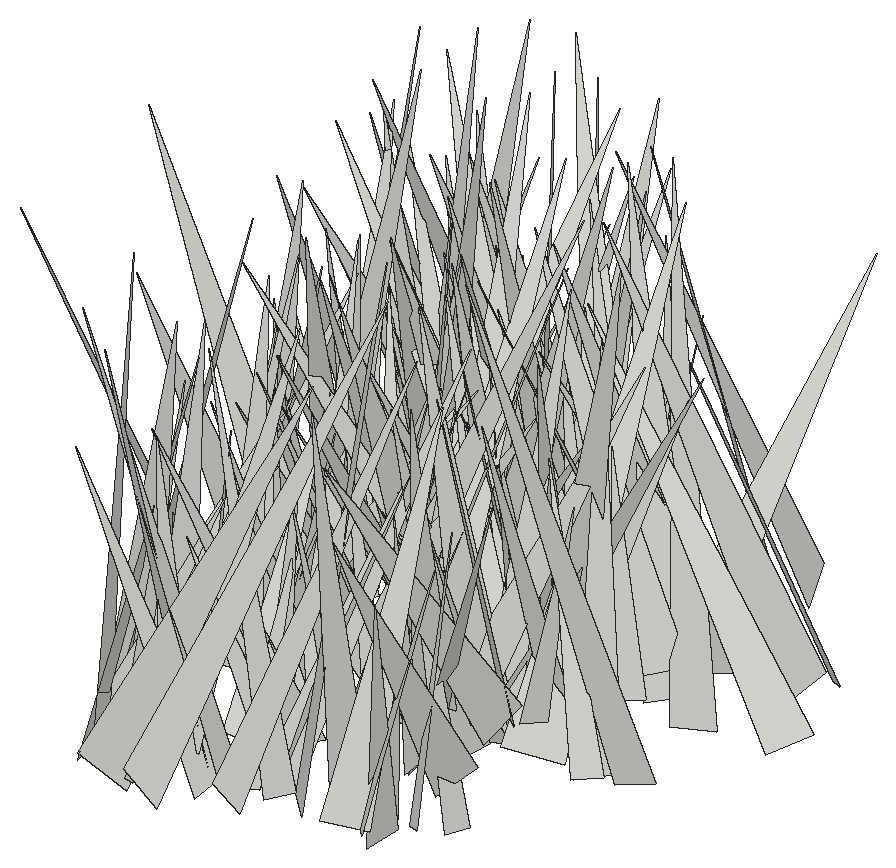
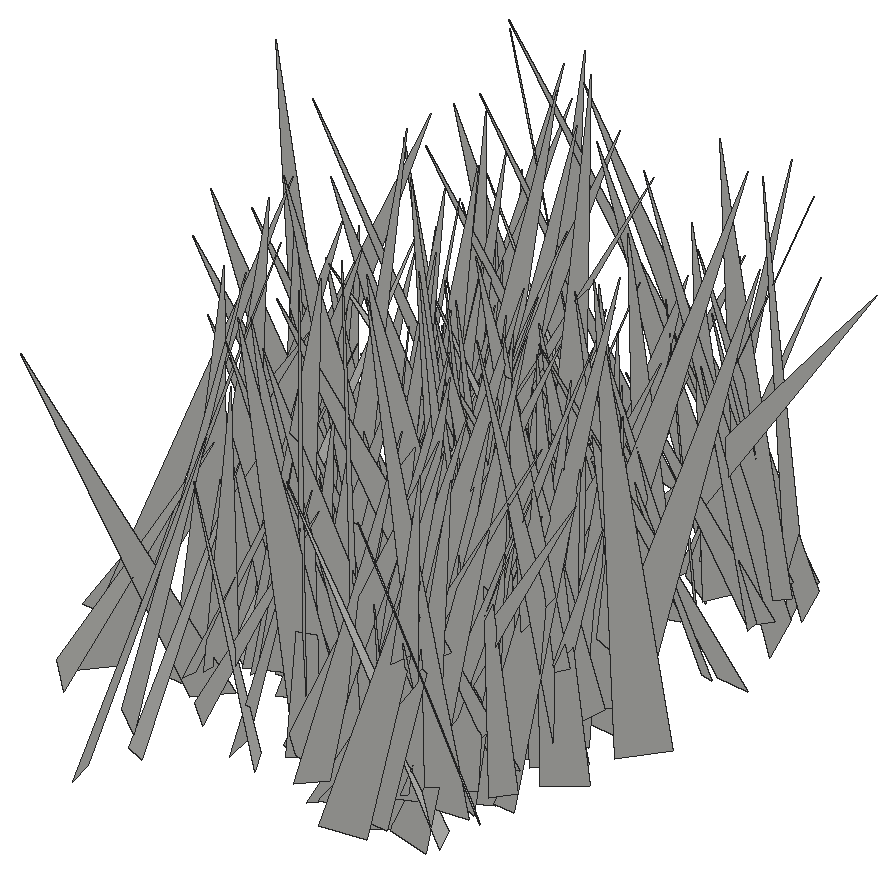
# SketchUp Ruby script. Lengths in inches.
U = 1.inch
M = Sketchup.active_model
def pt(a) = Geom::Point3d.new(a.map { |v| v * U })
def face(e, loops, mat)
  f = e.add_face(loops[0].map { |a| pt(a) })
  loops[1..].each { |l| e.add_face(l.map { |a| pt(a) }).erase! }
  f.material = f.back_material = mat if mat
  f
end
# faces: each face lists its corners as indices into pts; further lists are holes
def faces(e, pts, list, mat = nil) = list.each { |f| face(e, (f[0].is_a?(Array) ? f : [f]).map { |l| l.map { |i| pts[i] } }, mat) }
# xy, xz, yz: faces in a plane at the given z, y or x. An outline is a flat list of corners, or four numbers for a rectangle; further outlines are holes
def ring(l) = l.size == 4 ? [[l[0], l[1]], [l[2], l[1]], [l[2], l[3]], [l[0], l[3]]] : l.each_slice(2).to_a
def flat(e, list, mat, &to3) = list.each { |f| face(e, (f[0].is_a?(Array) ? f : [f]).map { |l| ring(l).map { |u, v| to3.(u, v) } }, mat) }
def xy(e, z, list, mat = nil) = flat(e, list, mat) { |x, y| [x, y, z] }
def xz(e, y, list, mat = nil) = flat(e, list, mat) { |x, z| [x, y, z] }
def yz(e, x, list, mat = nil) = flat(e, list, mat) { |y, z| [x, y, z] }
def lines(e, pts, list) = list.each { |a, b| e.add_line(pt(pts[a]), pt(pts[b])) }
# prism: a flat outline (further loops are holes) pulled along v
def prism(e, loops, v, mat = nil)
  f = face(e, loops, mat); d = Geom::Vector3d.new(v.map { |x| x * U })
  f.pushpull(f.normal.samedirection?(d) ? d.length : -d.length)
end
def box(e, o, s, mat = nil) = prism(e, [[o, [o[0] + s[0], o[1], o[2]], [o[0] + s[0], o[1] + s[1], o[2]], [o[0], o[1] + s[1], o[2]]]], [0, 0, s[2]], mat)
def at(x, y, z, deg = 0) = Geom::Transformation.translation(pt([x, y, z])) * Geom::Transformation.rotation(ORIGIN, Z_AXIS, deg.degrees)
def axes(o, x, y, z) = Geom::Transformation.new([*x, 0, *y, 0, *z, 0, *pt(o).to_a, 1])
def part(name) = M.definitions.add(name)
# library, detail: a bought-in or finely detailed component or shape, given as its bounding box
def library(name, o, s) = part(name).tap { |d| box(d.entities, o, s) }
def detail(e, o, s) = box(e.add_group.entities, o, s)
def put(e, d, t, mat = nil) = e.add_instance(d, t).tap { |i| i.material = mat if mat }
def group(e, t, mat = nil) = e.add_group.tap { |g| g.transformation = t; g.material = mat if mat }.entities
root = M.entities
c1 = part("fur_instance\#9")
p = [[0.8125,0,1.79],[0.67,-0.02,1.48],[0,-0.11,0],[0,0.11,0]]
faces(c1.entities,p,[[0,1,2,3]])
put(root,c1,axes([124.6,133.26,-27.1],[2.95346,-5.37759,1.21149],[-5.08452,-3.18852,-1.75785],[-2.12927,0.1548,5.87804]))
put(root,c1,axes([128.625,128.07,-27.1],[-5.00631,-5.98003,0.73957],[-5.22244,3.82659,-4.41068],[-3.00563,3.31169,6.43193]))
put(root,c1,axes([125.2,136.41,-28.22],[-4.0044,1.49429,0.5536],[1.5481,4.00291,0.3933],[0.37782,-0.56428,4.25599]))
put(root,c1,axes([122.98,134.41,-28.22],[5.02607,-4.57327,2.19343],[-4.92834,-5.13329,0.59007],[-1.19892,1.92923,6.76964]))
put(root,c1,axes([124.3,136.17,-27.1],[-6.72177,-1.11045,3.37602],[-2.29516,6.87097,-2.30972],[2.71346,3.06096,6.4094]))
put(root,c1,axes([123.3,140.08,-27.1],[3.09975,-1.98369,0.33098],[-1.98147,-3.11644,-0.1208],[-0.34401,0.07615,3.67817]))
put(root,c1,axes([123.22,141.34,-27.1],[3.32598,3.77438,0.4675],[3.78797,-3.34308,0.04133],[-0.34022,-0.32329,5.03054]))
put(root,c1,axes([124.6875,134.04,-28.22],[-0.34045,4.62028,2.07312],[5.05885,0.21591,0.34957],[-0.23002,-2.08976,4.6196]))
put(root,c1,axes([124.37,136.32,-28.22],[-3.77046,5.93467,2.17976],[6.06315,4.1134,-0.71146],[1.79161,-1.43096,6.99504]))
put(root,c1,axes([124.59,139.03,-28.22],[-0.43608,-7.58063,0.50958],[-7.59761,0.43802,0.01424],[0.04352,0.50791,7.59315]))
put(root,c1,axes([124.94,141.78,-27.1],[2.55776,-3.86723,2.22173],[-4.13899,-3.01226,-0.47827],[-1.66143,1.55064,4.61182]))
put(root,c1,axes([125.15,141.57,-27.1],[-6.3203,-1.31951,1.76492],[-0.3807,5.93404,3.07318],[2.17051,-2.80147,5.67828]))
put(root,c1,axes([126.85,132.5,-27.1],[-8.04315,1.60644,1.39343],[1.83623,7.99603,1.38066],[1.07265,-1.64234,8.08496]))
put(root,c1,axes([123.91,128.37,-27.1],[3.88682,0.49651,1.01606],[0.42112,-4.01087,0.34905],[-1.04955,0.22945,3.90283]))
put(root,c1,axes([124.9375,142.12,-28.22],[-2.01035,-7.12989,1.00319],[-7.18316,2.0575,0.22838],[0.49393,0.90254,7.40437]))
put(root,c1,axes([124.88,125.47,-28.22],[-6.34859,-2.07949,3.15929],[-2.7531,6.77324,-1.07409],[2.59343,2.09974,6.59357]))
put(root,c1,axes([124.9375,139.6875,-28.22],[-1.72033,-4.15588,1.09836],[-4.2769,1.77348,0.01157],[0.4311,1.01028,4.49785]))
put(root,c1,axes([127.28,139.64,-28.22],[-2.41735,-5.08882,0.8159],[-4.81582,1.90935,-2.35956],[-1.83565,1.69223,5.11586]))
put(root,c1,axes([123.05,131.6,-27.1],[2.48404,3.35431,0.63876],[3.34518,-2.23213,-1.28736],[0.685,-1.26336,3.97047]))
put(root,c1,axes([123.58,137.0625,-28.22],[3.13383,-5.16211,1.39491],[-5.34355,-3.08346,0.59403],[-0.19921,1.50298,6.00961]))
put(root,c1,axes([124.09,138.89,-27.1],[-0.30009,3.62925,0.24074],[3.53668,0.34756,-0.831],[0.84929,-0.16496,3.54556]))
put(root,c1,axes([125.05,139.48,-28.22],[3.99451,-5.40043,2.70776],[-5.64329,-4.49426,-0.63847],[-2.15638,1.75774,6.68679]))
put(root,c1,axes([125.58,134.85,-28.22],[-0.78367,4.54033,1.31363],[4.69244,0.5877,0.76808],[-0.56674,-1.41222,4.54299]))
put(root,c1,axes([125.78,141.83,-28.22],[-4.47005,3.93119,1.60818],[4.11701,4.5843,0.23722],[1.04438,-1.24571,5.94805]))
put(root,c1,axes([125.45,143.48,-27.1],[-0.22294,-7.81188,0.28991],[-7.80547,0.20653,-0.4373],[-0.42917,0.30182,7.80282]))
put(root,c1,axes([123.51,129.91,-28.22],[1.69788,6.23349,0.03172],[6.16311,-1.67374,-0.97718],[0.93461,-0.28707,6.38626]))
put(root,c1,axes([126.23,140.78,-28.22],[-3.87512,-3.17972,0.32504],[-3.163,3.88842,0.32938],[0.4601,-0.04943,5.00187]))
put(root,c1,axes([124.23,135.68,-27.1],[6.87844,-2.02965,2.77665],[-2.6588,-7.07628,1.41394],[-2.18175,2.22463,7.03088]))
put(root,c1,axes([125.39,144.39,-27.1],[2.94915,-5.28887,0.70098],[-5.06545,-3.02722,-1.5291],[-1.67475,-0.15728,5.85931]))
put(root,c1,axes([125.84,135.72,-27.1],[-1.40726,-4.75955,2.034],[-5.17479,1.24906,-0.65748],[-0.10975,2.13481,4.91949]))
put(root,c1,axes([125.1875,129.74,-27.1],[1.99951,5.4557,0.6063],[5.41529,-2.06607,0.73224],[-0.89823,-0.31139,5.76424]))
put(root,c1,axes([123.86,141.78,-27.1],[1.63751,6.97927,2.94123],[7.53115,-1.18196,-1.38823],[0.80173,-3.15202,7.03309]))
put(root,c1,axes([124.1,127.14,-28.22],[7.1658,2.76652,1.69463],[2.58302,-7.35112,1.0785],[-1.96302,0.42601,7.60521]))
put(root,c1,axes([123.96,133.4,-27.1],[5.74343,-0.59024,1.12729],[-0.57342,-5.85294,-0.14303],[-1.13593,-0.02976,5.77191]))
put(root,c1,axes([126.48,142.27,-27.1],[0.21554,-5.31829,2.18174],[-5.56977,-0.73327,-1.23719],[-1.42193,2.0661,5.17688]))
put(root,c1,axes([123.78,128.37,-27.1],[-0.24087,4.17753,0.95098],[3.88217,0.61574,-1.72155],[1.81241,-0.76371,3.81393]))
put(root,c1,axes([124.14,134.61,-27.1],[1.58205,-4.94043,0.08132],[-4.90313,-1.55912,0.66773],[0.6114,0.28046,5.1444]))
put(root,c1,axes([126.2,136.44,-27.1],[-1.47936,3.73163,0.54523],[3.76451,1.42617,0.45319],[-0.22551,-0.67216,3.98851]))
put(root,c1,axes([126.42,139.53,-28.22],[0.6459,3.9486,0.07217],[3.68247,-0.62859,1.43463],[-1.42692,0.16515,3.73504]))
put(root,c1,axes([124.57,125.24,-28.22],[5.61181,2.09612,1.30854],[1.89864,-5.73587,1.04566],[-1.58152,0.55181,5.89854]))
put(root,c1,axes([124.87,135.24,-28.22],[2.62732,-3.98087,0.28129],[-3.95197,-2.64215,-0.47983],[-0.55532,-0.03119,4.74551]))
put(root,c1,axes([128.1,141.75,-28.22],[-6.42762,0.7775,0.36666],[0.8533,6.10569,2.01137],[0.10407,-2.04186,6.15412]))
put(root,c1,axes([127.67,138.21,-28.22],[-6.07575,2.79462,0.62219],[2.80321,6.10345,-0.04049],[0.58225,-0.22305,6.68752]))
put(root,c1,axes([126.2,124.8,-28.22],[2.31766,5.02687,0.82298],[4.84651,-2.45447,1.34356],[-1.56781,-0.15629,5.3699]))
put(root,c1,axes([124.48,127.31,-27.1],[4.31409,-4.88001,1.43702],[-5.06352,-4.30068,0.59646],[-0.49016,1.47666,6.48614]))
put(root,c1,axes([124.49,140.625,-27.1],[6.011,-2.52803,0.45147],[-2.2406,-5.7244,-2.22212],[-1.25478,-1.8887,6.13068]))
put(root,c1,axes([125.58,138.38,-28.22],[3.41828,7.22194,2.57308],[7.56489,-3.63472,0.1519],[-1.24484,-2.25703,7.98861]))
put(root,c1,axes([125.49,127.78,-27.1],[-4.36102,2.95909,2.58691],[3.11538,4.95832,-0.41976],[2.39639,-1.06094,5.25343]))
put(root,c1,axes([126.96,140.57,-27.1],[1.83922,3.08635,0.93557],[2.6886,-2.06216,1.51739],[-1.78108,0.07419,3.25666]))
put(root,c1,axes([128.31,139.58,-28.22],[-5.45873,5.352,1.02249],[5.44819,5.38274,0.9113],[0.08123,-1.36725,7.5902]))
put(root,c1,axes([128.89,138.39,-27.1],[-6.43604,2.78332,0.65453],[2.85741,6.20344,1.71766],[-0.1023,-1.83529,6.79846]))
put(root,c1,axes([124.73,126.25,-27.1],[0.74077,3.76285,1.03817],[3.63302,-0.27816,-1.5841],[1.42759,-1.24465,3.49262]))
put(root,c1,axes([126.09,140.55,-27.1],[4.34994,-4.04005,0.73934],[-3.73736,-4.34022,-1.72779],[-1.70317,-0.79441,5.67968]))
put(root,c1,axes([126.73,140.62,-28.22],[-0.19276,-5.01478,1.27598],[-5.16585,0.1124,-0.33865],[-0.30027,1.28555,5.00705]))
put(root,c1,axes([126.15,129.83,-27.1],[-1.18817,5.57554,2.26119],[5.96275,1.39894,-0.31626],[0.80332,-2.13721,5.69196]))
put(root,c1,axes([128.11,135.02,-28.22],[-4.21104,-1.2398,0.43934],[-1.31531,3.95873,-1.43574],[-0.00925,1.50143,4.14832]))
put(root,c1,axes([124.22,141.47,-28.22],[4.96423,2.67259,0.04648],[2.6631,-4.93667,-0.5706],[0.22978,-0.52435,5.60898]))
put(root,c1,axes([128.35,125.78,-28.22],[-5.33847,-0.05884,0.40473],[-0.0096,5.31499,0.64603],[0.40887,-0.64342,5.29956]))
put(root,c1,axes([128.78,141.92,-27.1],[-0.87207,-5.64239,2.10409],[-5.67136,0.05471,-2.20385],[-2.02471,2.277,5.26688]))
put(root,c1,axes([127.5625,126.44,-28.22],[-3.47477,-5.64058,1.59223],[-5.83486,3.50381,-0.32112],[0.55295,1.52727,6.61718]))
put(root,c1,axes([129.53,125.15,-27.1],[-6.43064,-2.17008,0.24743],[-2.17262,6.27662,-1.4168],[-0.22404,1.42068,6.6374]))
put(root,c1,axes([126.78,126.42,-27.1],[2.27684,-3.73592,1.683],[-3.94498,-2.51908,-0.25488],[-1.10756,1.29258,4.36763]))
put(root,c1,axes([126.21,128.06,-28.22],[3.53151,3.08583,1.68165],[3.37882,-3.63698,-0.42174],[-0.96639,-1.43941,4.67077]))
put(root,c1,axes([127.87,140.97,-27.1],[-1.21907,-3.82959,1.50139],[-4.09681,0.98993,-0.80143],[-0.36895,1.66143,3.93822]))
put(root,c1,axes([127.8,142.71,-27.1],[-5.01187,1.13995,1.85475],[1.60842,5.07616,1.22637],[1.46717,-1.67079,4.99142]))
put(root,c1,axes([128.38,128.99,-28.22],[1.26657,4.59176,1.22685],[4.36989,-1.62436,1.56816],[-1.86909,-0.68616,4.4977]))
put(root,c1,axes([128.57,133.68,-28.22],[0.11807,-5.18176,0.38422],[-4.95689,-0.22756,-1.54584],[-1.55804,0.33133,4.94722]))
put(root,c1,axes([127.53,141.59,-28.22],[3.87648,-5.20572,1.47803],[-5.00062,-4.14086,-1.46909],[-2.0683,0.2548,6.32205]))
put(root,c1,axes([126.36,132.26,-27.1],[-1.839,3.01934,1.93742],[3.07994,2.44517,-0.88715],[1.83955,-1.07548,3.42218]))
put(root,c1,axes([125.93,130.49,-28.22],[2.61371,2.45973,0.53308],[2.49517,-2.43181,-1.01309],[0.32949,-1.09634,3.44317]))
put(root,c1,axes([128.46,130.32,-27.1],[-4.34148,-1.68145,0.56308],[-1.64517,4.37512,0.38015],[0.66161,-0.1544,4.64018]))
put(root,c1,axes([125.98,138.34,-27.1],[7.89082,-0.9052,1.78608],[-0.78265,-8.07818,-0.63641],[-1.84308,-0.44515,7.91703]))
put(root,c1,axes([128.9,129.51,-27.1],[0.42359,6.38348,0.10104],[6.1795,-0.43539,1.60081],[-1.60398,0.00839,6.194]))
put(root,c1,axes([126.625,133.3,-28.22],[3.82826,-1.89723,1.31218],[-2.241,-3.66166,1.2438],[-0.54703,1.72325,4.08754]))
put(root,c1,axes([127.24,129.99,-28.22],[4.20313,-0.16718,1.34956],[-0.39887,-4.34286,0.70427],[-1.30006,0.79192,4.14708]))
put(root,c1,axes([126.3,134.15,-27.1],[7.64117,-3.1953,0.94942],[-2.87226,-7.51641,-2.18001],[-1.69158,-1.67105,7.9903]))
put(root,c1,axes([128.42,136.83,-28.22],[3.29752,4.92899,1.52703],[4.76096,-3.60504,1.35547],[-1.98997,-0.45731,5.77332]))
put(root,c1,axes([128.33,137.96,-27.1],[-3.06281,-3.15709,1.43812],[-3.29391,3.24851,0.11628],[1.08883,0.94666,4.3971]))
put(root,c1,axes([124.9,131.96,-28.22],[2.725,5.40327,0.30402],[4.86473,-2.29653,-2.78814],[2.3711,-1.498,5.37096]))
put(root,c1,axes([130.17,127.86,-27.1],[0.21984,-5.04241,1.33274],[-4.72838,-0.75562,-2.0789],[-2.20101,1.11963,4.59917]))
put(root,c1,axes([129.04,134.98,-28.22],[-4.17954,-4.03403,0.06779],[-3.83281,4.00041,1.74723],[1.26,-1.21235,5.53978]))
put(root,c1,axes([128.56,126.875,-27.1],[-0.5351,4.97369,0.08314],[4.96853,0.53845,-0.2337],[0.24128,-0.05757,4.99693]))
put(root,c1,axes([127.36,125.7,-27.1],[0.34617,6.42334,1.62872],[6.51894,-0.03728,-1.2385],[1.18972,-1.66468,6.31231]))
put(root,c1,axes([127.24,135.32,-28.22],[-1.37451,8.097,0.63904],[7.82187,1.49419,-2.10823],[2.18815,-0.25501,7.93763]))
put(root,c1,axes([131.4,125.07,-27.1],[0.1109,6.16383,0.84068],[5.38265,-0.51661,3.07768],[-3.11876,-0.67243,5.34163]))
put(root,c1,axes([130.1,132.34,-28.22],[-5.1626,-2.88411,0.4563],[-2.82641,5.16852,0.6903],[0.7333,-0.3834,5.87316]))
put(root,c1,axes([126.76,136.29,-28.22],[3.85978,2.30102,0.3483],[2.28006,-3.60384,-1.45862],[0.46617,-1.42533,4.2503]))
put(root,c1,axes([128.1,137.46,-28.22],[0.00091,-3.67707,1.93886],[-4.08733,0.35251,0.67045],[0.75747,1.90654,3.61543]))
put(root,c1,axes([125.58,124.68,-28.22],[0.25719,7.17904,2.90731],[6.91163,1.10018,-3.3281],[3.49578,-2.70337,6.36621]))
put(root,c1,axes([128.66,132.8,-28.22],[-5.68198,1.58826,2.45655],[1.00817,6.10119,-1.61279],[2.74605,1.04639,5.67506]))
put(root,c1,axes([129.1,139.08,-28.22],[6.18055,4.14964,3.19418],[4.26505,-6.85588,0.65402],[-3.03836,-1.18276,7.41558]))
put(root,c1,axes([127.84,140.45,-27.1],[-0.91329,-6.82842,0.06821],[-6.63421,0.90353,1.6239],[1.61843,-0.14959,6.69511]))
put(root,c1,axes([129.83,126.8125,-27.1],[-3.46593,0.7925,0.89611],[1.04093,3.35143,1.06213],[0.58952,-1.25841,3.39303]))
put(root,c1,axes([129.92,134.32,-27.1],[-5.97227,4.9002,0.90124],[4.6479,5.98621,-1.7477],[1.79477,0.80344,7.52499]))
put(root,c1,axes([129.53,137.54,-28.22],[-5.63617,-2.55407,1.20627],[-1.85262,5.37498,2.72438],[2.13217,-2.08115,5.55585]))
put(root,c1,axes([129.58,133.09,-27.1],[-5.36603,-1.88935,2.74168],[-2.67241,5.54565,-1.40882],[1.98613,2.35731,5.51173]))
put(root,c1,axes([127.95,138.72,-28.22],[6.10707,-2.19869,2.10682],[-2.76305,-5.98564,1.76265],[-1.28003,2.43046,6.24689]))
put(root,c1,axes([129.14,126.38,-28.22],[-2.50227,2.59124,1.1484],[2.47228,2.74461,-0.80603],[1.38608,-0.21748,3.51087]))
put(root,c1,axes([129.06,127.78,-27.1],[0.06663,3.86387,1.64805],[4.18879,0.06273,-0.31643],[0.31563,-1.6482,3.85147]))
put(root,c1,axes([130.43,130.59,-28.22],[-0.54656,4.2534,1.19948],[4.32093,0.26075,1.04426],[-0.92722,-1.29209,4.15928]))
put(root,c1,axes([129.59,140.875,-27.1],[4.46233,4.90899,2.88894],[5.22756,-4.98695,0.39938],[-2.26203,-1.84084,6.62202]))
put(root,c1,axes([128.83,141.8,-27.1],[2.48728,-3.44318,0.65298],[-3.47724,-2.52444,-0.0662],[-0.43662,0.49004,4.24707]))
put(root,c1,axes([129.43,134.65,-28.22],[0.59961,-8.00132,0.48644],[-8.01433,-0.60861,-0.13198],[-0.1682,0.47514,8.02267]))
put(root,c1,axes([128.24,133.86,-28.22],[-1.2496,-4.95098,2.04852],[-4.91628,1.89585,1.58307],[2.13046,1.47094,4.85465]))
put(root,c1,axes([132.71,134.02,-28.22],[-8.10416,-1.22815,0.06312],[-1.16757,7.81624,2.17553],[0.38615,-2.14192,7.90272]))
put(root,c1,axes([129.2,140.57,-27.1],[-3.21117,5.73542,2.2751],[5.803,3.67883,-1.08356],[2.09673,-1.39782,6.48325]))
put(root,c1,axes([127.61,134.66,-27.1],[1.13497,4.33314,1.68645],[4.04549,-0.06445,-2.557],[2.29221,-2.03177,3.67778]))
put(root,c1,axes([132.34,138.58,-27.1],[-4.81407,6.51041,0.79127],[6.55623,4.75265,0.78417],[-0.16528,-1.10168,8.05889]))
put(root,c1,axes([132.68,131.65,-27.1],[-5.08452,-4.09315,0.88657],[-4.17476,4.84247,-1.58557],[-0.33349,1.78573,6.33184]))
put(root,c1,axes([131.3,135.02,-28.22],[-4.54367,3.48057,1.82928],[3.81076,4.58683,0.73803],[0.96889,-1.71821,5.67579]))
put(root,c1,axes([129.38,138.7,-27.1],[1.31333,6.20143,0.89],[6.24264,-1.21867,-0.72041],[0.52849,-1.01577,6.2979]))
put(root,c1,axes([131.75,140.92,-28.22],[-4.57594,-0.69447,0.70937],[-0.73517,4.61906,-0.2203],[0.6671,0.32667,4.62309]))
put(root,c1,axes([130.01,134.5,-28.22],[6.29678,-5.28708,1.00032],[-4.88133,-6.26054,-2.36253],[-2.26416,-1.20654,7.87535]))
put(root,c1,axes([128.36,136.57,-28.22],[3.7348,-2.45498,0.02516],[-2.33086,-3.53122,1.44009],[0.77113,1.21649,4.23106]))
put(root,c1,axes([131.72,127.85,-28.22],[-1.05409,-4.02831,1.60299],[-4.27873,0.70037,-1.05356],[-0.69957,1.78611,4.02845]))
put(root,c1,axes([128.19,123.04,-27.1],[3.14457,7.68443,0.45621],[7.56933,-2.99688,-1.69436],[1.40136,-1.05601,8.12822]))
put(root,c1,axes([132.49,141.72,-27.1],[-2.45002,-3.17903,0.27674],[-3.09062,2.27713,-1.20338],[-0.79426,0.94543,3.82893]))
put(root,c1,axes([129.99,139.55,-27.1],[5.84499,-0.86217,1.83487],[-1.09003,-6.05756,0.62599],[-1.70936,0.91471,5.87498]))
put(root,c1,axes([130.42,131.75,-28.22],[0.78552,4.64999,1.51438],[4.88897,-0.70993,-0.35606],[0.11721,-1.55126,4.70241]))
put(root,c1,axes([130.8125,136.06,-27.1],[2.01145,-6.31603,1.30369],[-6.40118,-2.12156,-0.40211],[-0.78536,1.11557,6.61638]))
put(root,c1,axes([132.23,137.82,-28.22],[-4.35819,2.96505,1.59627],[3.3258,4.19926,1.28011],[0.52792,-1.97688,5.11338]))
put(root,c1,axes([130.49,138.79,-27.1],[7.53052,-1.13144,2.64431],[-0.30654,-7.68469,-2.41514],[-2.85982,-2.15562,7.22191]))
put(root,c1,axes([131.94,136.72,-28.22],[-3.91317,-2.34388,0.53173],[-2.28614,3.94348,0.55853],[0.74167,-0.21123,4.52711]))
put(root,c1,axes([132.65,138.4375,-27.1],[-5.52094,1.92393,0.48296],[1.85996,5.5174,-0.71721],[0.68943,0.52184,5.80241]))
put(root,c1,axes([129.18,136.43,-28.22],[7.2049,-3.47591,1.96261],[-3.83046,-7.15988,1.38131],[-1.1231,2.12096,7.87937]))
put(root,c1,axes([132.23,134.56,-27.1],[-2.23276,3.13779,0.67741],[3.20125,2.1153,0.75324],[-0.23799,-0.9847,3.77672]))
put(root,c1,axes([130.43,128.99,-27.1],[4.1336,3.03674,0.5342],[2.87698,-4.11997,1.15876],[-1.10914,0.6308,4.99657]))
put(root,c1,axes([132.42,133.72,-27.1],[-3.36159,2.04077,0.19725],[2.04893,3.35754,0.1809],[0.07444,-0.25709,3.9284]))
put(root,c1,axes([130.5,132.13,-27.1],[-1.86477,7.56726,1.18834],[7.49142,2.05683,-1.34204],[1.5982,-0.81177,7.67722]))
put(root,c1,axes([132.6,132.47,-28.22],[0.06912,-7.57158,0.2529],[-7.42195,-0.11839,-1.51598],[-1.51902,0.23392,7.41859]))
put(root,c1,axes([131.92,137.49,-27.1],[-1.38179,3.78074,1.32931],[4.00762,1.30133,0.46468],[-0.00636,-1.40818,3.99842]))
put(root,c1,axes([132.16,136.13,-27.1],[-3.20539,-1.99252,1.2784],[-2.28309,3.17085,-0.78241],[0.62603,1.36182,3.69222]))
put(root,c1,axes([130.61,136.82,-28.22],[-3.46675,-5.54657,1.13696],[-5.08588,3.63649,2.23277],[2.48816,-0.29493,6.14797]))
put(root,c1,axes([130.87,141.22,-28.22],[-3.23487,-1.73884,2.61208],[-2.22596,3.91581,-0.14997],[2.2117,1.39779,3.66954]))
put(root,c1,axes([131.73,131.44,-28.22],[-3.10303,1.40825,1.48641],[1.65077,3.31728,0.3033],[1.21143,-0.91317,3.39411]))
put(root,c1,axes([132.57,133.97,-28.22],[-4.62696,-2.40171,1.71965],[-2.7299,4.69747,-0.78458],[1.12828,1.51649,5.15378]))
put(root,c1,axes([129.13,131.41,-27.1],[3.76818,7.24013,0.96766],[7.17608,-3.46602,-2.01138],[1.36373,-1.76699,7.91031]))
put(root,c1,axes([132.28,132.98,-28.22],[4.49335,-4.83843,2.48866],[-4.8443,-5.0271,-1.02712],[-2.47721,1.05444,6.5227]))
put(root,c1,axes([131.52,128.26,-28.22],[5.70548,5.18554,0.14342],[4.71826,-5.27598,3.06024],[-2.15603,2.1765,7.07653]))
put(root,c1,axes([130.36,124.04,-27.1],[2.81698,6.47491,0.35167],[6.46114,-2.77024,-0.75032],[0.54938,-0.62035,7.02117]))
put(root,c1,axes([130.69,126.08,-27.1],[1.99959,6.47326,0.24716],[6.43471,-1.95494,-0.85747],[0.74746,-0.48749,6.72058]))
put(root,c1,axes([132.1,125,-27.1],[5.36611,5.59511,2.05394],[5.5109,-5.71038,1.15783],[-2.27022,-0.63666,7.66549]))
put(root,c1,axes([130.46,126.27,-27.1],[4.29759,3.17988,0.45483],[3.21134,-4.23507,-0.73441],[0.07624,-0.86047,5.29543]))
put(root,c1,axes([131.91,132.9,-28.22],[2.51881,-4.55482,0.15905],[-4.51842,-2.51942,-0.59372],[-0.59628,-0.14918,5.17091]))
put(root,c1,axes([133.73,138.48,-27.1],[-4.47092,-4.93614,0.16266],[-4.90041,4.46105,0.68268],[0.61475,-0.33851,6.62484]))
put(root,c1,axes([133.125,133.34,-28.22],[-3.70308,-3.24105,0.05421],[-3.08159,3.54543,1.46762],[1.00557,-1.07036,4.69716]))
put(root,c1,axes([132.5,133.28,-27.1],[-0.07417,5.83715,1.21265],[5.95855,0.11247,-0.17697],[0.19614,-1.2097,5.83493]))
put(root,c1,axes([131.5,136.92,-27.1],[5.7747,-1.11479,0.95698],[-0.77258,-5.60537,-1.86777],[-1.24967,-1.68603,5.57685]))
put(root,c1,axes([133.84,139.08,-27.1],[-5.20641,1.3754,0.94823],[1.21962,5.25029,-0.91901],[1.14166,0.66356,5.30602]))
put(root,c1,axes([133.74,143.22,-27.1],[-4.39451,-5.32367,1.29551],[-5.40377,4.48556,0.10243],[0.905,0.93264,6.90237]))
put(root,c1,axes([132.7,131.54,-28.22],[5.55902,-2.83125,1.90418],[-2.404,-5.83322,-1.65498],[-2.42129,-0.70867,6.01496]))
put(root,c1,axes([134.04,140.19,-27.1],[-4.91943,-1.92287,0.32626],[-1.70701,4.67316,1.80343],[0.9434,-1.57124,4.96446]))
put(root,c1,axes([134.2,144.72,-28.22],[-7.22673,-3.69522,1.05519],[-3.3656,7.17065,2.06111],[1.85494,-1.38592,7.85061]))
put(root,c1,axes([133,126.15,-27.1],[0.27233,-6.25887,1.87066],[-6.53155,-0.29195,-0.02597],[-0.1084,1.8677,6.26474]))
put(root,c1,axes([133.22,128.59,-27.1],[3.59976,0.06174,1.80471],[0.19659,-4.01441,-0.2548],[-1.79504,-0.31584,3.59126]))
put(root,c1,axes([133.38,132.42,-27.1],[-3.17607,-4.40082,1.193],[-4.40846,3.33508,0.56622],[1.16445,0.62283,5.3976]))
put(root,c1,axes([135.17,136.85,-27.1],[-3.75455,5.21199,1.89568],[5.51913,3.28609,1.89629],[-0.5456,-2.62523,6.13723]))
put(root,c1,axes([132.36,130.55,-27.1],[5.38586,-3.00561,1.16634],[-2.8404,-5.49795,-1.05176],[-1.52519,-0.37466,6.07741]))
put(root,c1,axes([135.09,128.1,-28.22],[-5.0928,-0.09663,0.30052],[-0.16718,4.94609,-1.24277],[0.26777,1.25023,4.93978]))
put(root,c1,axes([133.74,142.91,-28.22],[-2.1706,-3.79382,0.07549],[-3.76138,2.16267,0.53397],[0.50075,-0.20018,4.33814]))
put(root,c1,axes([132.875,127.88,-28.22],[-1.15878,-4.12917,1.68532],[-4.31214,1.48176,0.66553],[1.13832,1.40977,4.23673]))
put(root,c1,axes([133.07,137.05,-28.22],[0.22863,4.55848,1.01522],[4.65358,-0.13679,-0.43379],[0.39321,-1.03161,4.54355]))
put(root,c1,axes([133.65,131.86,-27.1],[5.96418,-2.86813,1.57613],[-1.66285,-5.47776,-3.67572],[-2.81874,-2.83722,5.50334]))
put(root,c1,axes([134.96,139.11,-28.22],[1.43067,-7.01564,1.7352],[-6.90944,-1.84641,-1.76845],[-2.11892,1.28394,6.9382]))
put(root,c1,axes([134.23,133.58,-27.1],[-0.19346,-4.85951,0.89963],[-4.92735,0.1202,-0.41034],[-0.38132,0.91231,4.84602]))
put(root,c1,axes([132.68,134.14,-28.22],[1.98838,-4.24744,1.75797],[-4.57109,-1.62434,1.24561],[0.4862,2.09896,4.52138]))
put(root,c1,axes([135.11,137.51,-28.22],[-5.88987,4.84378,2.23578],[5.14185,6.04195,0.45575],[1.42207,-1.78441,7.61217]))
put(root,c1,axes([131.5,132.23,-28.22],[0.86928,6.52033,1.58307],[6.24969,-0.2059,-2.58369],[2.44176,-1.79425,6.04937]))
put(root,c1,axes([133.78,124.89,-27.1],[-3.09006,5.24053,1.65653],[5.13422,3.43055,-1.27548],[1.9614,-0.72379,5.94851]))
put(root,c1,axes([131.89,130.69,-28.22],[6.41369,-0.07562,0.05633],[-0.05586,-6.13403,-1.87481],[-0.07597,-1.87412,6.13403]))
put(root,c1,axes([134.07,132.63,-28.22],[-3.86216,7.0455,1.20437],[6.7899,4.04407,-1.88376],[2.2331,-0.11104,7.81068]))
put(root,c1,axes([132.78,134.98,-28.22],[0.51844,5.23573,1.343],[5.13497,-0.0558,-1.76472],[1.68777,-1.43851,4.95655]))
put(root,c1,axes([136.55,136.46,-28.22],[-0.02832,7.80203,1.3013],[7.5934,-0.33756,2.1891],[-2.2148,-1.25708,7.48868]))
put(root,c1,axes([133.78,126.52,-28.22],[4.60045,-1.39498,0.802],[-1.20201,-4.59424,-1.0961],[-1.06973,-0.83684,4.68067]))
put(root,c1,axes([135.3,125.94,-27.1],[2.28996,3.33239,0.84649],[3.03653,-2.43723,1.38011],[-1.61271,0.14282,3.80053]))
put(root,c1,axes([134.22,132.51,-27.1],[3.08181,-1.73974,0.98019],[-1.88437,-3.1302,0.36886],[-0.66077,0.81254,3.51969]))
put(root,c1,axes([132.32,133.57,-28.22],[6.21247,-1.9108,0.54363],[-1.98453,-5.88708,1.9863],[0.09123,2.05733,6.18874]))
put(root,c1,axes([134.17,125.08,-27.1],[2.95956,2.83712,0.75066],[2.89518,-2.997,-0.08741],[-0.48027,-0.58351,4.09885]))
put(root,c1,axes([134.63,128.66,-27.1],[5.34512,-3.23236,0.64666],[-2.65449,-4.95104,-2.80671],[-1.95449,-2.11559,5.5804]))
put(root,c1,axes([135.48,135.09,-27.1],[-2.21806,2.84038,1.31516],[3.07662,2.27502,0.2754],[0.57601,-1.21396,3.59328]))
put(root,c1,axes([133.36,134.82,-27.1],[1.45469,-7.67033,1.86376],[-7.74266,-1.0178,1.85445],[1.53584,2.13396,7.5836]))
put(root,c1,axes([138,140.83,-28.22],[-3.48224,-3.77241,0.29956],[-3.58403,3.15695,-1.90663],[-1.21472,1.49981,4.76674]))
put(root,c1,axes([136.18,132.81,-28.22],[-5.32179,3.05618,1.70346],[3.04909,5.5718,-0.47069],[1.71611,-0.42222,6.11884]))
put(root,c1,axes([134.125,139.08,-28.22],[-1.13308,6.40977,0.66119],[6.08836,1.28481,-2.02171],[2.11049,-0.26515,6.18722]))
put(root,c1,axes([139.1,137.43,-28.22],[-4.14935,5.21761,0.66717],[4.85978,3.47746,3.02911],[-2.01273,-2.35998,5.93844]))
put(root,c1,axes([137.53,139.93,-28.22],[-7.8024,0.71377,1.7229],[1.19599,7.6017,2.26696],[1.43089,-2.46171,7.49986]))
put(root,c1,axes([138.46,131.57,-27.1],[-0.67807,6.71445,3.30984],[6.96597,-0.65101,2.74773],[-2.74118,-3.31527,6.16389]))
put(root,c1,axes([137.26,131,-27.1],[-1.4583,4.1794,0.64732],[4.14586,1.27741,1.09233],[-0.83566,-0.95598,4.28962]))
